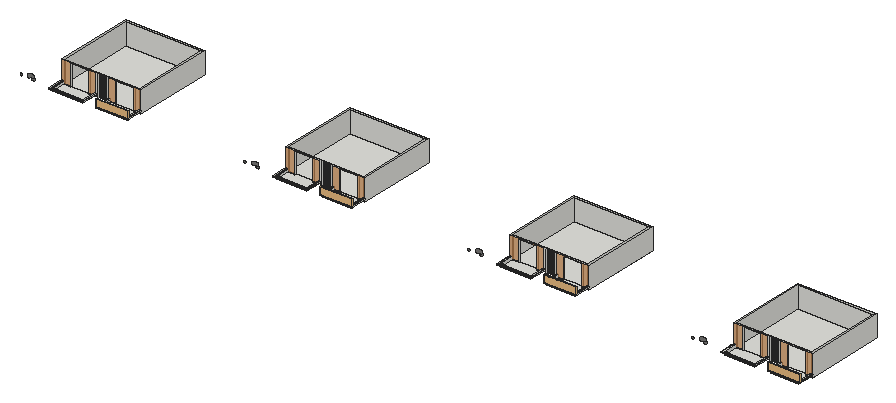
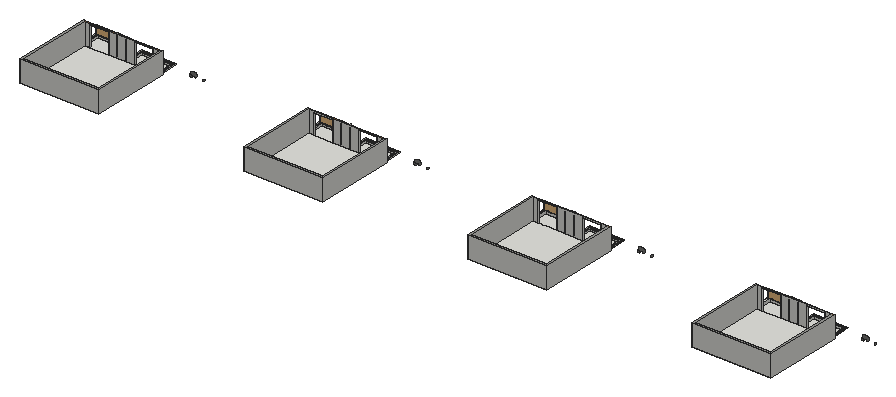
# SketchUp Ruby script. Lengths in inches.
U = 1.inch
M = Sketchup.active_model
def pt(a) = Geom::Point3d.new(a.map { |v| v * U })
def face(e, loops, mat)
  f = e.add_face(loops[0].map { |a| pt(a) })
  loops[1..].each { |l| e.add_face(l.map { |a| pt(a) }).erase! }
  f.material = f.back_material = mat if mat
  f
end
# faces: each face lists its corners as indices into pts; further lists are holes
def faces(e, pts, list, mat = nil) = list.each { |f| face(e, (f[0].is_a?(Array) ? f : [f]).map { |l| l.map { |i| pts[i] } }, mat) }
# xy, xz, yz: faces in a plane at the given z, y or x. An outline is a flat list of corners, or four numbers for a rectangle; further outlines are holes
def ring(l) = l.size == 4 ? [[l[0], l[1]], [l[2], l[1]], [l[2], l[3]], [l[0], l[3]]] : l.each_slice(2).to_a
def flat(e, list, mat, &to3) = list.each { |f| face(e, (f[0].is_a?(Array) ? f : [f]).map { |l| ring(l).map { |u, v| to3.(u, v) } }, mat) }
def xy(e, z, list, mat = nil) = flat(e, list, mat) { |x, y| [x, y, z] }
def xz(e, y, list, mat = nil) = flat(e, list, mat) { |x, z| [x, y, z] }
def yz(e, x, list, mat = nil) = flat(e, list, mat) { |y, z| [x, y, z] }
def lines(e, pts, list) = list.each { |a, b| e.add_line(pt(pts[a]), pt(pts[b])) }
# prism: a flat outline (further loops are holes) pulled along v
def prism(e, loops, v, mat = nil)
  f = face(e, loops, mat); d = Geom::Vector3d.new(v.map { |x| x * U })
  f.pushpull(f.normal.samedirection?(d) ? d.length : -d.length)
end
def box(e, o, s, mat = nil) = prism(e, [[o, [o[0] + s[0], o[1], o[2]], [o[0] + s[0], o[1] + s[1], o[2]], [o[0], o[1] + s[1], o[2]]]], [0, 0, s[2]], mat)
def at(x, y, z, deg = 0) = Geom::Transformation.translation(pt([x, y, z])) * Geom::Transformation.rotation(ORIGIN, Z_AXIS, deg.degrees)
def axes(o, x, y, z) = Geom::Transformation.new([*x, 0, *y, 0, *z, 0, *pt(o).to_a, 1])
def part(name) = M.definitions.add(name)
# library, detail: a bought-in or finely detailed component or shape, given as its bounding box
def library(name, o, s) = part(name).tap { |d| box(d.entities, o, s) }
def detail(e, o, s) = box(e.add_group.entities, o, s)
def put(e, d, t, mat = nil) = e.add_instance(d, t).tap { |i| i.material = mat if mat }
def group(e, t, mat = nil) = e.add_group.tap { |g| g.transformation = t; g.material = mat if mat }.entities
root = M.entities
M.materials.add("[0043_SaddleBrown]4").color = [124, 123, 122]
M.materials.add("[Granite Light Gray]").color = [149, 148, 144]
M.materials.add("[Wood Floor]").color = [224, 152, 88]
M.materials["[Wood Floor]"].alpha = 0.68
c1 = library("Glass Railing",[0,0,0],[139.5,4.76,42])
xy(root,526.4375,[[563.08,570.83,734.59,570.83,734.59,651.03,703.26,651.03,703.26,657.03,602.01,657.03,602.01,651.03,563.08,651.03],[820.97,570.83,978.86,570.83,978.86,651.03,951.01,651.03,951.01,657.03,849.76,657.03,849.76,651.03,820.97,651.03],[1813.71,570.83,1985.21,570.83,1985.21,651.03,1953.89,651.03,1953.89,657.03,1852.64,657.03,1852.64,651.03,1813.71,651.03],[2071.59,570.83,2229.49,570.83,2229.49,651.03,2201.63,651.03,2201.63,657.03,2100.38,657.03,2100.38,651.03,2071.59,651.03],[3064.33,570.83,3235.84,570.83,3235.84,651.03,3204.51,651.03,3204.51,657.03,3103.26,657.03,3103.26,651.03,3064.33,651.03],
  [3322.22,570.83,3480.11,570.83,3480.11,651.03,3452.26,651.03,3452.26,657.03,3351.01,657.03,3351.01,651.03,3322.22,651.03],[4314.96,570.83,4486.46,570.83,4486.46,651.03,4455.14,651.03,4455.14,657.03,4353.89,657.03,4353.89,651.03,4314.96,651.03],[4572.84,570.83,4730.74,570.83,4730.74,651.03,4702.88,651.03,4702.88,657.03,4601.63,657.03,4601.63,651.03,4572.84,651.03],[551.76,651.03,551.76,1096.5,990.19,1096.5,990.19,651.03,951.01,651.03,951.01,657.03,978.86,657.03,978.86,1085.17,563.08,1085.17,563.08,657.03,602.01,657.03,602.01,651.03],[1802.38,651.03,1802.38,1096.5,2240.81,1096.5,2240.81,651.03,2201.63,651.03,2201.63,657.03,2229.49,657.03,2229.49,1085.17,1813.71,1085.17,1813.71,657.03,1852.64,657.03,1852.64,651.03],
  [3053.01,651.03,3053.01,1096.5,3491.44,1096.5,3491.44,651.03,3452.26,651.03,3452.26,657.03,3480.11,657.03,3480.11,1085.17,3064.33,1085.17,3064.33,657.03,3103.26,657.03,3103.26,651.03],[4303.63,651.03,4303.63,1096.5,4742.06,1096.5,4742.06,651.03,4702.88,651.03,4702.88,657.03,4730.74,657.03,4730.74,1085.17,4314.96,1085.17,4314.96,657.03,4353.89,657.03,4353.89,651.03],[563.08,657.03,978.86,1085.17],[1813.71,657.03,2229.49,1085.17],[3064.33,657.03,3480.11,1085.17],
  [4314.96,657.03,4730.74,1085.17]])
xy(root,538.1875,[[550.01,558.125,742.44,559.875],[742.44,558.125,744.19,647.91],[814.68,558.125,991.94,559.875],[1800.63,558.125,1993.07,559.875],[1993.07,558.125,1994.82,647.91],
  [2065.31,558.125,2242.56,559.875],[3051.26,558.125,3243.69,559.875],[3243.69,558.125,3245.44,647.91],[3315.93,558.125,3493.19,559.875],[4301.88,558.125,4494.32,559.875],
  [4494.32,558.125,4496.07,647.91],[4566.56,558.125,4743.81,559.875],[550.01,559.875,551.76,640.11],[551.76,559.875,551.76,651.03,563.08,651.03,563.08,570.83,734.59,570.83,734.59,651.03,742.44,651.03,742.44,559.875],[814.68,559.875,814.89,651.03],
  [814.89,559.875,814.89,651.03,820.97,651.03,820.97,570.83,978.86,570.83,978.86,651.03,990.19,651.03,990.19,559.875],[990.19,559.875,991.94,651.03],[1800.63,559.875,1802.38,640.11],[1802.38,559.875,1802.38,651.03,1813.71,651.03,1813.71,570.83,1985.21,570.83,1985.21,651.03,1993.07,651.03,1993.07,559.875],[2065.31,559.875,2065.52,651.03],
  [2065.52,559.875,2065.52,651.03,2071.59,651.03,2071.59,570.83,2229.49,570.83,2229.49,651.03,2240.81,651.03,2240.81,559.875],[2240.81,559.875,2242.56,651.03],[3051.26,559.875,3053.01,640.11],[3053.01,559.875,3053.01,651.03,3064.33,651.03,3064.33,570.83,3235.84,570.83,3235.84,651.03,3243.69,651.03,3243.69,559.875],[3315.93,559.875,3316.14,651.03],
  [3316.14,559.875,3316.14,651.03,3322.22,651.03,3322.22,570.83,3480.11,570.83,3480.11,651.03,3491.44,651.03,3491.44,559.875],[3491.44,559.875,3493.19,651.03],[4301.88,559.875,4303.63,640.11],[4303.63,559.875,4303.63,651.03,4314.96,651.03,4314.96,570.83,4486.46,570.83,4486.46,651.03,4494.32,651.03,4494.32,559.875],[4566.56,559.875,4566.77,651.03],
  [4566.77,559.875,4566.77,651.03,4572.84,651.03,4572.84,570.83,4730.74,570.83,4730.74,651.03,4742.06,651.03,4742.06,559.875],[4742.06,559.875,4743.81,651.03]])
xz(root,558.125,[[550.01,538.1875,744.19,541.1875],[814.68,538.1875,991.94,541.1875],[1800.63,538.1875,1994.82,541.1875],[2065.31,538.1875,2242.56,541.1875],[3051.26,538.1875,3245.44,541.1875],
  [3315.93,538.1875,3493.19,541.1875],[4301.88,538.1875,4496.07,541.1875],[4566.56,538.1875,4743.81,541.1875]],"[Granite Light Gray]")
xz(root,570.83,[[563.08,526.4375,734.59,538.1875],[820.97,526.4375,978.86,538.1875],[1813.71,526.4375,1985.21,538.1875],[2071.59,526.4375,2229.49,538.1875],[3064.33,526.4375,3235.84,538.1875],
  [3322.22,526.4375,3480.11,538.1875],[4314.96,526.4375,4486.46,538.1875],[4572.84,526.4375,4730.74,538.1875],[563.08,538.1875,734.59,541.1875],[820.97,538.1875,978.86,541.1875],
  [1813.71,538.1875,1985.21,541.1875],[2071.59,538.1875,2229.49,541.1875],[3064.33,538.1875,3235.84,541.1875],[3322.22,538.1875,3480.11,541.1875],[4314.96,538.1875,4486.46,541.1875],
  [4572.84,538.1875,4730.74,541.1875]])
xz(root,589.17,[[437.09,527.94,436.99,528.61,436.83,529.26,436.62,529.92,436.35,530.5625,436.03,531.2,435.66,531.82,435.23,532.4375,434.76,533.04,434.24,533.62,433.67,534.18,433.05,534.73,432.39,535.26,434.04,535.17,435.7,535.18,437.35,535.3,438.98,535.51,440.55,535.83,442.07,536.25,443.51,536.76,444.86,537.35,446.1,538.03,447.23,538.78,448.22,539.6,449.07,540.47,449.07,529.79,448.03,529.77,447,529.73,445.96,529.66,444.9375,529.57,443.92,529.45,442.9,529.31,441.9,529.14,440.91,528.95,439.93,528.73,438.97,528.49,438.02,528.23],[1687.72,527.94,1687.61,528.61,1687.45,529.26,1687.24,529.92,1686.97,530.5625,1686.65,531.2,1686.28,531.82,1685.86,532.4375,1685.38,533.04,1684.86,533.62,1684.29,534.18,1683.68,534.73,1683.01,535.26,1684.67,535.17,1686.33,535.18,1687.98,535.3,1689.6,535.51,1691.18,535.83,1692.7,536.25,1694.14,536.76,1695.48,537.35,1696.73,538.03,1697.85,538.78,1698.84,539.6,1699.7,540.47,1699.7,529.79,1698.66,529.77,1697.62,529.73,1696.59,529.66,1695.5625,529.57,1694.54,529.45,1693.53,529.31,1692.53,529.14,1691.53,528.95,1690.56,528.73,1689.59,528.49,1688.65,528.23],[2938.34,527.94,2938.24,528.61,2938.08,529.26,2937.87,529.92,2937.6,530.5625,2937.28,531.2,2936.91,531.82,2936.48,532.4375,2936.01,533.04,2935.49,533.62,2934.92,534.18,2934.3,534.73,2933.64,535.26,2935.29,535.17,2936.95,535.18,2938.6,535.3,2940.23,535.51,2941.8,535.83,2943.32,536.25,2944.76,536.76,2946.11,537.35,2947.35,538.03,2948.48,538.78,2949.47,539.6,2950.32,540.47,2950.32,529.79,2949.28,529.77,2948.25,529.73,2947.21,529.66,2946.1875,529.57,2945.17,529.45,2944.15,529.31,2943.15,529.14,2942.16,528.95,2941.18,528.73,2940.22,528.49,2939.27,528.23],[4188.97,527.94,4188.86,528.61,4188.7,529.26,4188.49,529.92,4188.22,530.5625,4187.9,531.2,4187.53,531.82,4187.11,532.4375,4186.63,533.04,4186.11,533.62,4185.54,534.18,4184.93,534.73,4184.26,535.26,4185.92,535.17,4187.58,535.18,4189.23,535.3,4190.85,535.51,4192.43,535.83,4193.95,536.25,4195.39,536.76,4196.73,537.35,4197.98,538.03,4199.1,538.78,4200.09,539.6,4200.95,540.47,4200.95,529.79,4199.91,529.77,4198.87,529.73,4197.84,529.66,4196.8125,529.57,4195.79,529.45,4194.78,529.31,4193.78,529.14,4192.78,528.95,4191.81,528.73,4190.84,528.49,4189.9,528.23],[376.03,530.76,375.33,530.98,374.64,531.21,373.97,531.47,373.31,531.73,372.67,532.01,372.05,532.3,371.44,532.61,370.85,532.93,370.28,533.26,369.73,533.6,369.19,533.95,368.68,534.32,368.68,540.38,369.2,539.84,369.79,539.33,370.45,538.84,371.17,538.39,371.94,537.98,372.77,537.61,373.65,537.28,374.5625,537,375.51,536.76,376.49,536.57,377.49,536.43,378.51,536.35,378.09,535.93,377.71,535.5,377.36,535.06,377.05,534.6,376.78,534.14,376.55,533.67,376.36,533.19,376.21,532.71,376.11,532.23,376.04,531.74,376.01,531.25],
  [1626.65,530.76,1625.95,530.98,1625.27,531.21,1624.6,531.47,1623.94,531.73,1623.3,532.01,1622.67,532.3,1622.07,532.61,1621.48,532.93,1620.9,533.26,1620.35,533.6,1619.82,533.95,1619.31,534.32,1619.31,540.38,1619.83,539.84,1620.42,539.33,1621.07,538.84,1621.79,538.39,1622.57,537.98,1623.4,537.61,1624.27,537.28,1625.1875,537,1626.14,536.76,1627.12,536.57,1628.12,536.43,1629.13,536.35,1628.71,535.93,1628.33,535.5,1627.99,535.06,1627.68,534.6,1627.41,534.14,1627.18,533.67,1626.99,533.19,1626.84,532.71,1626.73,532.23,1626.66,531.74,1626.64,531.25],[2877.28,530.76,2876.58,530.98,2875.89,531.21,2875.22,531.47,2874.56,531.73,2873.92,532.01,2873.3,532.3,2872.69,532.61,2872.1,532.93,2871.53,533.26,2870.98,533.6,2870.44,533.95,2869.93,534.32,2869.93,540.38,2870.45,539.84,2871.04,539.33,2871.7,538.84,2872.42,538.39,2873.19,537.98,2874.02,537.61,2874.9,537.28,2875.8125,537,2876.76,536.76,2877.74,536.57,2878.74,536.43,2879.76,536.35,2879.34,535.93,2878.96,535.5,2878.61,535.06,2878.3,534.6,2878.03,534.14,2877.8,533.67,2877.61,533.19,2877.46,532.71,2877.36,532.23,2877.29,531.74,2877.26,531.25],[4127.9,530.76,4127.2,530.98,4126.52,531.21,4125.85,531.47,4125.19,531.73,4124.55,532.01,4123.92,532.3,4123.32,532.61,4122.73,532.93,4122.15,533.26,4121.6,533.6,4121.07,533.95,4120.56,534.32,4120.56,540.38,4121.08,539.84,4121.67,539.33,4122.32,538.84,4123.04,538.39,4123.82,537.98,4124.65,537.61,4125.52,537.28,4126.4375,537,4127.39,536.76,4128.37,536.57,4129.37,536.43,4130.38,536.35,4129.96,535.93,4129.58,535.5,4129.24,535.06,4128.93,534.6,4128.66,534.14,4128.43,533.67,4128.24,533.19,4128.09,532.71,4127.98,532.23,4127.91,531.74,4127.89,531.25],[416.47,534.48,415.35,535.4,414.34,536.36,413.45,537.37,412.6875,538.42,412.05,539.49,411.55,540.6,411.18,541.72,410.95,542.86,410.85,544.01,410.9,545.15,411.08,546.29,411.4,547.42,411.93,548.64,412.66,549.82,413.59,550.95,414.69,552.01,415.97,553,417.4,553.91,418.97,554.72,420.67,555.42,422.48,556.02,424.38,556.5,426.35,556.86,428.37,557.1,430.57,557.19,432.77,557.1,434.93,556.82,437.01,556.37,438.97,555.75,440.78,554.97,442.39,554.04,443.79,552.99,444.9375,551.84,445.82,550.59,446.42,549.29,446.73,547.95,446.72,546.78,446.4375,545.63,445.88,544.52,445.07,543.46,444.02,542.5,442.74,541.63,441.28,540.89,439.65,540.29,437.9,539.85,436.0625,539.56,434.17,539.44,432.28,539.5,430.81,539.68,429.4,540.01,428.11,540.48,426.95,541.07,425.97,541.77,425.1875,542.56,424.625,543.42,424.3,544.32,424.22,545.24,424.39,546.16,424.79,547.05,425.43,547.88,425.95,548.22,426.56,548.48,427.26,548.66,428,548.75,428.75,548.75,429.48,548.65,430.17,548.46,430.77,548.19,431.28,547.84,431.66,547.44,431.89,547,431.78,546.7,431.72,546.4,431.72,546.09,431.77,545.78,431.88,545.48,432.04,545.1875,432.26,544.91,432.52,544.65,432.84,544.4,433.19,544.18,433.58,543.99,434.01,543.83,435.02,543.91,435.99,544.1,436.91,544.37,437.75,544.73,438.49,545.16,439.12,545.65,439.61,546.2,439.96,546.79,440.16,547.41,440.21,548.03,440.09,548.66,439.82,549.26,439.08,550.27,438.07,551.1875,436.82,551.99,435.375,552.66,433.77,553.16,432.05,553.5,430.26,553.65,428.45,553.625,426.68,553.41,424.99,553.01,423.4375,552.45,422.05,551.74,420.6,550.73,419.38,549.62,418.41,548.41,417.7,547.14,417.27,545.82,417.125,544.48,417.27,543.14,417.7,541.82,418.41,540.55,419.38,539.34,420.6,538.23,422.05,537.22,421.69,536.92,421.31,536.64,420.9,536.36,420.48,536.1,420.03,535.85,419.57,535.61,419.09,535.39,418.6,535.18,418.09,534.98,417.5625,534.8,417.02,534.63],[1667.1,534.48,1665.98,535.4,1664.97,536.36,1664.08,537.37,1663.3125,538.42,1662.68,539.49,1662.17,540.6,1661.8,541.72,1661.57,542.86,1661.48,544.01,1661.52,545.15,1661.71,546.29,1662.03,547.42,1662.56,548.64,1663.29,549.82,1664.21,550.95,1665.32,552.01,1666.59,553,1668.02,553.91,1669.6,554.72,1671.3,555.42,1673.11,556.02,1675.01,556.5,1676.97,556.86,1678.99,557.1,1681.2,557.19,1683.4,557.1,1685.56,556.82,1687.64,556.37,1689.6,555.75,1691.4,554.97,1693.02,554.04,1694.41,552.99,1695.5625,551.84,1696.45,550.59,1697.05,549.29,1697.35,547.95,1697.35,546.78,1697.0625,545.63,1696.51,544.52,1695.7,543.46,1694.64,542.5,1693.37,541.63,1691.9,540.89,1690.28,540.29,1688.52,539.85,1686.6875,539.56,1684.8,539.44,1682.9,539.5,1681.43,539.68,1680.03,540.01,1678.73,540.48,1677.58,541.07,1676.59,541.77,1675.8125,542.56,1675.25,543.42,1674.93,544.32,1674.84,545.24,1675.01,546.16,1675.42,547.05,1676.06,547.88,1676.57,548.22,1677.19,548.48,1677.88,548.66,1678.62,548.75,1679.37,548.75,1680.11,548.65,1680.79,548.46,1681.4,548.19,1681.9,547.84,1682.28,547.44,1682.52,547,1682.4,546.7,1682.34,546.4,1682.34,546.09,1682.4,545.78,1682.5,545.48,1682.67,545.1875,1682.88,544.91,1683.15,544.65,1683.46,544.4,1683.82,544.18,1684.21,543.99,1684.63,543.83,1685.64,543.91,1686.62,544.1,1687.54,544.37,1688.38,544.73,1689.12,545.16,1689.74,545.65,1690.24,546.2,1690.59,546.79,1690.79,547.41,1690.83,548.03,1690.72,548.66,1690.45,549.26,1689.7,550.27,1688.69,551.1875,1687.45,551.99,1686,552.66,1684.39,553.16,1682.67,553.5,1680.89,553.65,1679.08,553.625,1677.31,553.41,1675.62,553.01,1674.0625,552.45,1672.68,551.74,1671.23,550.73,1670.01,549.62,1669.03,548.41,1668.32,547.14,1667.9,545.82,1667.75,544.48,1667.9,543.14,1668.32,541.82,1669.03,540.55,1670.01,539.34,1671.23,538.23,1672.68,537.22,1672.32,536.92,1671.93,536.64,1671.53,536.36,1671.1,536.1,1670.66,535.85,1670.2,535.61,1669.72,535.39,1669.22,535.18,1668.71,534.98,1668.1875,534.8,1667.65,534.63],
  [2917.72,534.48,2916.6,535.4,2915.59,536.36,2914.7,537.37,2913.9375,538.42,2913.3,539.49,2912.8,540.6,2912.43,541.72,2912.2,542.86,2912.1,544.01,2912.15,545.15,2912.33,546.29,2912.65,547.42,2913.18,548.64,2913.91,549.82,2914.84,550.95,2915.94,552.01,2917.22,553,2918.65,553.91,2920.22,554.72,2921.92,555.42,2923.73,556.02,2925.63,556.5,2927.6,556.86,2929.62,557.1,2931.82,557.19,2934.02,557.1,2936.18,556.82,2938.26,556.37,2940.22,555.75,2942.03,554.97,2943.64,554.04,2945.04,552.99,2946.1875,551.84,2947.07,550.59,2947.67,549.29,2947.98,547.95,2947.97,546.78,2947.6875,545.63,2947.13,544.52,2946.32,543.46,2945.27,542.5,2943.99,541.63,2942.53,540.89,2940.9,540.29,2939.15,539.85,2937.3125,539.56,2935.42,539.44,2933.53,539.5,2932.06,539.68,2930.65,540.01,2929.36,540.48,2928.2,541.07,2927.22,541.77,2926.4375,542.56,2925.875,543.42,2925.55,544.32,2925.47,545.24,2925.64,546.16,2926.04,547.05,2926.68,547.88,2927.2,548.22,2927.81,548.48,2928.51,548.66,2929.25,548.75,2930,548.75,2930.73,548.65,2931.42,548.46,2932.02,548.19,2932.53,547.84,2932.91,547.44,2933.14,547,2933.03,546.7,2932.97,546.4,2932.97,546.09,2933.02,545.78,2933.13,545.48,2933.29,545.1875,2933.51,544.91,2933.77,544.65,2934.09,544.4,2934.44,544.18,2934.83,543.99,2935.26,543.83,2936.27,543.91,2937.24,544.1,2938.16,544.37,2939,544.73,2939.74,545.16,2940.37,545.65,2940.86,546.2,2941.21,546.79,2941.41,547.41,2941.46,548.03,2941.34,548.66,2941.07,549.26,2940.33,550.27,2939.32,551.1875,2938.07,551.99,2936.625,552.66,2935.02,553.16,2933.3,553.5,2931.51,553.65,2929.7,553.625,2927.93,553.41,2926.24,553.01,2924.6875,552.45,2923.3,551.74,2921.85,550.73,2920.63,549.62,2919.66,548.41,2918.95,547.14,2918.52,545.82,2918.375,544.48,2918.52,543.14,2918.95,541.82,2919.66,540.55,2920.63,539.34,2921.85,538.23,2923.3,537.22,2922.94,536.92,2922.56,536.64,2922.15,536.36,2921.73,536.1,2921.28,535.85,2920.82,535.61,2920.34,535.39,2919.85,535.18,2919.34,534.98,2918.8125,534.8,2918.27,534.63],[4168.35,534.48,4167.23,535.4,4166.22,536.36,4165.33,537.37,4164.5625,538.42,4163.93,539.49,4163.42,540.6,4163.05,541.72,4162.82,542.86,4162.73,544.01,4162.77,545.15,4162.96,546.29,4163.28,547.42,4163.81,548.64,4164.54,549.82,4165.46,550.95,4166.57,552.01,4167.84,553,4169.27,553.91,4170.85,554.72,4172.55,555.42,4174.36,556.02,4176.26,556.5,4178.22,556.86,4180.24,557.1,4182.45,557.19,4184.65,557.1,4186.81,556.82,4188.89,556.37,4190.85,555.75,4192.65,554.97,4194.27,554.04,4195.66,552.99,4196.8125,551.84,4197.7,550.59,4198.3,549.29,4198.6,547.95,4198.6,546.78,4198.3125,545.63,4197.76,544.52,4196.95,543.46,4195.89,542.5,4194.62,541.63,4193.15,540.89,4191.53,540.29,4189.77,539.85,4187.9375,539.56,4186.05,539.44,4184.15,539.5,4182.68,539.68,4181.28,540.01,4179.98,540.48,4178.83,541.07,4177.84,541.77,4177.0625,542.56,4176.5,543.42,4176.18,544.32,4176.09,545.24,4176.26,546.16,4176.67,547.05,4177.31,547.88,4177.82,548.22,4178.44,548.48,4179.13,548.66,4179.87,548.75,4180.62,548.75,4181.36,548.65,4182.04,548.46,4182.65,548.19,4183.15,547.84,4183.53,547.44,4183.77,547,4183.65,546.7,4183.59,546.4,4183.59,546.09,4183.65,545.78,4183.75,545.48,4183.92,545.1875,4184.13,544.91,4184.4,544.65,4184.71,544.4,4185.07,544.18,4185.46,543.99,4185.88,543.83,4186.89,543.91,4187.87,544.1,4188.79,544.37,4189.63,544.73,4190.37,545.16,4190.99,545.65,4191.49,546.2,4191.84,546.79,4192.04,547.41,4192.08,548.03,4191.97,548.66,4191.7,549.26,4190.95,550.27,4189.94,551.1875,4188.7,551.99,4187.25,552.66,4185.64,553.16,4183.92,553.5,4182.14,553.65,4180.33,553.625,4178.56,553.41,4176.87,553.01,4175.3125,552.45,4173.93,551.74,4172.48,550.73,4171.26,549.62,4170.28,548.41,4169.57,547.14,4169.15,545.82,4169,544.48,4169.15,543.14,4169.57,541.82,4170.28,540.55,4171.26,539.34,4172.48,538.23,4173.93,537.22,4173.57,536.92,4173.18,536.64,4172.78,536.36,4172.35,536.1,4171.91,535.85,4171.45,535.61,4170.97,535.39,4170.47,535.18,4169.96,534.98,4169.4375,534.8,4168.9,534.63]],"[0043_SaddleBrown]4")
xz(root,640.11,[[550.01,538.1875,551.76,541.1875],[1800.63,538.1875,1802.38,541.1875],[3051.26,538.1875,3053.01,541.1875],[4301.88,538.1875,4303.63,541.1875]])
xz(root,647.91,[[742.44,538.1875,744.19,541.1875],[1993.07,538.1875,1994.82,541.1875],[3243.69,538.1875,3245.44,541.1875],[4494.32,538.1875,4496.07,541.1875]])
xz(root,651.03,[[551.76,526.4375,563.08,538.1875],[978.86,526.4375,990.19,538.1875],[1802.38,526.4375,1813.71,538.1875],[2229.49,526.4375,2240.81,538.1875],[3053.01,526.4375,3064.33,538.1875],
  [3480.11,526.4375,3491.44,538.1875],[4303.63,526.4375,4314.96,538.1875],[4730.74,526.4375,4742.06,538.1875],[551.76,538.1875,563.08,541.1875],[734.59,538.1875,742.44,541.1875],
  [814.68,538.1875,820.97,541.1875],[978.86,538.1875,990.19,541.1875],[990.19,538.1875,991.94,541.1875],[1802.38,538.1875,1813.71,541.1875],[1985.21,538.1875,1993.07,541.1875],
  [2065.31,538.1875,2071.59,541.1875],[2229.49,538.1875,2240.81,541.1875],[2240.81,538.1875,2242.56,541.1875],[3053.01,538.1875,3064.33,541.1875],[3235.84,538.1875,3243.69,541.1875],
  [3315.93,538.1875,3322.22,541.1875],[3480.11,538.1875,3491.44,541.1875],[3491.44,538.1875,3493.19,541.1875],[4303.63,538.1875,4314.96,541.1875],[4486.46,538.1875,4494.32,541.1875],
  [4566.56,538.1875,4572.84,541.1875],[4730.74,538.1875,4742.06,541.1875],[4742.06,538.1875,4743.81,541.1875]])
xz(root,651.03,[[563.08,526.4375,602.01,526.4375,602.01,640.875,703.26,640.875,703.26,526.4375,734.59,526.4375,734.59,541.1875,742.44,541.1875,742.44,646.4375,551.76,646.4375,551.76,541.1875,563.08,541.1875],[820.97,526.4375,849.76,526.4375,849.76,640.875,951.01,640.875,951.01,526.4375,978.86,526.4375,978.86,541.1875,990.19,541.1875,990.19,646.4375,814.89,646.4375,814.89,541.1875,820.97,541.1875],[1813.71,526.4375,1852.64,526.4375,1852.64,640.875,1953.89,640.875,1953.89,526.4375,1985.21,526.4375,1985.21,541.1875,1993.07,541.1875,1993.07,646.4375,1802.38,646.4375,1802.38,541.1875,1813.71,541.1875],[2071.59,526.4375,2100.38,526.4375,2100.38,640.875,2201.63,640.875,2201.63,526.4375,2229.49,526.4375,2229.49,541.1875,2240.81,541.1875,2240.81,646.4375,2065.52,646.4375,2065.52,541.1875,2071.59,541.1875],[3064.33,526.4375,3103.26,526.4375,3103.26,640.875,3204.51,640.875,3204.51,526.4375,3235.84,526.4375,3235.84,541.1875,3243.69,541.1875,3243.69,646.4375,3053.01,646.4375,3053.01,541.1875,3064.33,541.1875],
  [3322.22,526.4375,3351.01,526.4375,3351.01,640.875,3452.26,640.875,3452.26,526.4375,3480.11,526.4375,3480.11,541.1875,3491.44,541.1875,3491.44,646.4375,3316.14,646.4375,3316.14,541.1875,3322.22,541.1875],[4314.96,526.4375,4353.89,526.4375,4353.89,640.875,4455.14,640.875,4455.14,526.4375,4486.46,526.4375,4486.46,541.1875,4494.32,541.1875,4494.32,646.4375,4303.63,646.4375,4303.63,541.1875,4314.96,541.1875],[4572.84,526.4375,4601.63,526.4375,4601.63,640.875,4702.88,640.875,4702.88,526.4375,4730.74,526.4375,4730.74,541.1875,4742.06,541.1875,4742.06,646.4375,4566.77,646.4375,4566.77,541.1875,4572.84,541.1875]],"[Wood Floor]")
xz(root,657.03,[[563.08,526.4375,563.08,646.4375,978.86,646.4375,978.86,526.4375,951.01,526.4375,951.01,640.875,849.76,640.875,849.76,526.4375,703.26,526.4375,703.26,640.875,602.01,640.875,602.01,526.4375],[1813.71,526.4375,1813.71,646.4375,2229.49,646.4375,2229.49,526.4375,2201.63,526.4375,2201.63,640.875,2100.38,640.875,2100.38,526.4375,1953.89,526.4375,1953.89,640.875,1852.64,640.875,1852.64,526.4375],[3064.33,526.4375,3064.33,646.4375,3480.11,646.4375,3480.11,526.4375,3452.26,526.4375,3452.26,640.875,3351.01,640.875,3351.01,526.4375,3204.51,526.4375,3204.51,640.875,3103.26,640.875,3103.26,526.4375],[4314.96,526.4375,4314.96,646.4375,4730.74,646.4375,4730.74,526.4375,4702.88,526.4375,4702.88,640.875,4601.63,640.875,4601.63,526.4375,4455.14,526.4375,4455.14,640.875,4353.89,640.875,4353.89,526.4375]])
xz(root,1085.17,[[563.08,526.4375,978.86,646.4375],[1813.71,526.4375,2229.49,646.4375],[3064.33,526.4375,3480.11,646.4375],[4314.96,526.4375,4730.74,646.4375]])
xz(root,1096.5,[[551.76,526.4375,990.19,646.4375],[1802.38,526.4375,2240.81,646.4375],[3053.01,526.4375,3491.44,646.4375],[4303.63,526.4375,4742.06,646.4375]])
yz(root,550.01,[[558.125,538.1875,640.11,541.1875]])
yz(root,551.76,[[651.03,526.4375,1096.5,646.4375],[640.11,538.1875,651.03,541.1875]])
yz(root,563.08,[[570.83,526.4375,651.03,538.1875],[657.03,526.4375,1085.17,646.4375],[570.83,538.1875,651.03,541.1875]])
yz(root,602.01,[[651.03,526.4375,657.03,640.875]])
yz(root,703.26,[[651.03,526.4375,657.03,640.875]])
yz(root,734.59,[[570.83,526.4375,651.03,538.1875],[570.83,538.1875,651.03,541.1875]])
yz(root,742.44,[[647.91,538.1875,651.03,541.1875]])
yz(root,744.19,[[558.125,538.1875,647.91,541.1875]])
yz(root,755.44,[[647.91,526.4375,651.03,646.4375]])
yz(root,768.19,[[648.85,526.4375,651.03,646.4375]])
yz(root,780.32,[[648.85,526.4375,651.03,646.4375]])
yz(root,792.69,[[648.85,526.4375,651.03,646.4375]])
yz(root,805.57,[[648.85,526.4375,651.03,646.4375]])
yz(root,814.68,[[558.125,538.1875,648.85,541.1875],[648.85,538.1875,651.03,541.1875]])
yz(root,820.97,[[570.83,526.4375,651.03,538.1875],[570.83,538.1875,651.03,541.1875]])
yz(root,849.76,[[651.03,526.4375,657.03,640.875]])
yz(root,951.01,[[651.03,526.4375,657.03,640.875]])
yz(root,978.86,[[570.83,526.4375,651.03,538.1875],[657.03,526.4375,1085.17,646.4375],[570.83,538.1875,651.03,541.1875]])
yz(root,990.19,[[651.03,526.4375,1096.5,646.4375]])
yz(root,991.94,[[558.125,538.1875,651.03,541.1875]])
yz(root,1800.63,[[558.125,538.1875,640.11,541.1875]])
yz(root,1802.38,[[651.03,526.4375,1096.5,646.4375],[640.11,538.1875,651.03,541.1875]])
yz(root,1813.71,[[570.83,526.4375,651.03,538.1875],[657.03,526.4375,1085.17,646.4375],[570.83,538.1875,651.03,541.1875]])
yz(root,1852.64,[[651.03,526.4375,657.03,640.875]])
yz(root,1953.89,[[651.03,526.4375,657.03,640.875]])
yz(root,1985.21,[[570.83,526.4375,651.03,538.1875],[570.83,538.1875,651.03,541.1875]])
yz(root,1993.07,[[647.91,538.1875,651.03,541.1875]])
yz(root,1994.82,[[558.125,538.1875,647.91,541.1875]])
yz(root,2006.07,[[647.91,526.4375,651.03,646.4375]])
yz(root,2018.82,[[648.85,526.4375,651.03,646.4375]])
yz(root,2030.94,[[648.85,526.4375,651.03,646.4375]])
yz(root,2043.32,[[648.85,526.4375,651.03,646.4375]])
yz(root,2056.19,[[648.85,526.4375,651.03,646.4375]])
yz(root,2065.31,[[558.125,538.1875,648.85,541.1875],[648.85,538.1875,651.03,541.1875]])
yz(root,2071.59,[[570.83,526.4375,651.03,538.1875],[570.83,538.1875,651.03,541.1875]])
yz(root,2100.38,[[651.03,526.4375,657.03,640.875]])
yz(root,2201.63,[[651.03,526.4375,657.03,640.875]])
yz(root,2229.49,[[570.83,526.4375,651.03,538.1875],[657.03,526.4375,1085.17,646.4375],[570.83,538.1875,651.03,541.1875]])
yz(root,2240.81,[[651.03,526.4375,1096.5,646.4375]])
yz(root,2242.56,[[558.125,538.1875,651.03,541.1875]])
yz(root,3051.26,[[558.125,538.1875,640.11,541.1875]])
yz(root,3053.01,[[651.03,526.4375,1096.5,646.4375],[640.11,538.1875,651.03,541.1875]])
yz(root,3064.33,[[570.83,526.4375,651.03,538.1875],[657.03,526.4375,1085.17,646.4375],[570.83,538.1875,651.03,541.1875]])
yz(root,3103.26,[[651.03,526.4375,657.03,640.875]])
yz(root,3204.51,[[651.03,526.4375,657.03,640.875]])
yz(root,3235.84,[[570.83,526.4375,651.03,538.1875],[570.83,538.1875,651.03,541.1875]])
yz(root,3243.69,[[647.91,538.1875,651.03,541.1875]])
yz(root,3245.44,[[558.125,538.1875,647.91,541.1875]])
yz(root,3256.69,[[647.91,526.4375,651.03,646.4375]])
yz(root,3269.44,[[648.85,526.4375,651.03,646.4375]])
yz(root,3281.57,[[648.85,526.4375,651.03,646.4375]])
yz(root,3293.94,[[648.85,526.4375,651.03,646.4375]])
yz(root,3306.82,[[648.85,526.4375,651.03,646.4375]])
yz(root,3315.93,[[558.125,538.1875,648.85,541.1875],[648.85,538.1875,651.03,541.1875]])
yz(root,3322.22,[[570.83,526.4375,651.03,538.1875],[570.83,538.1875,651.03,541.1875]])
yz(root,3351.01,[[651.03,526.4375,657.03,640.875]])
yz(root,3452.26,[[651.03,526.4375,657.03,640.875]])
yz(root,3480.11,[[570.83,526.4375,651.03,538.1875],[657.03,526.4375,1085.17,646.4375],[570.83,538.1875,651.03,541.1875]])
yz(root,3491.44,[[651.03,526.4375,1096.5,646.4375]])
yz(root,3493.19,[[558.125,538.1875,651.03,541.1875]])
yz(root,4301.88,[[558.125,538.1875,640.11,541.1875]])
yz(root,4303.63,[[651.03,526.4375,1096.5,646.4375],[640.11,538.1875,651.03,541.1875]])
yz(root,4314.96,[[570.83,526.4375,651.03,538.1875],[657.03,526.4375,1085.17,646.4375],[570.83,538.1875,651.03,541.1875]])
yz(root,4353.89,[[651.03,526.4375,657.03,640.875]])
yz(root,4455.14,[[651.03,526.4375,657.03,640.875]])
yz(root,4486.46,[[570.83,526.4375,651.03,538.1875],[570.83,538.1875,651.03,541.1875]])
yz(root,4494.32,[[647.91,538.1875,651.03,541.1875]])
yz(root,4496.07,[[558.125,538.1875,647.91,541.1875]])
yz(root,4507.32,[[647.91,526.4375,651.03,646.4375]])
yz(root,4520.07,[[648.85,526.4375,651.03,646.4375]])
yz(root,4532.19,[[648.85,526.4375,651.03,646.4375]])
yz(root,4544.57,[[648.85,526.4375,651.03,646.4375]])
yz(root,4557.44,[[648.85,526.4375,651.03,646.4375]])
yz(root,4566.56,[[558.125,538.1875,648.85,541.1875],[648.85,538.1875,651.03,541.1875]])
yz(root,4572.84,[[570.83,526.4375,651.03,538.1875],[570.83,538.1875,651.03,541.1875]])
yz(root,4601.63,[[651.03,526.4375,657.03,640.875]])
yz(root,4702.88,[[651.03,526.4375,657.03,640.875]])
yz(root,4730.74,[[570.83,526.4375,651.03,538.1875],[657.03,526.4375,1085.17,646.4375],[570.83,538.1875,651.03,541.1875]])
yz(root,4742.06,[[651.03,526.4375,1096.5,646.4375]])
yz(root,4743.81,[[558.125,538.1875,651.03,541.1875]])
put(root,c1,axes([3315.93,559.875,538.1875],[1.2691,0,0],[0,1,0],[0,0,1]))
put(root,c1,axes([4566.56,559.875,538.1875],[1.2691,0,0],[0,1,0],[0,0,1]))
put(root,c1,axes([814.68,559.875,538.1875],[1.2691,0,0],[0,1,0],[0,0,1]))
put(root,c1,axes([2065.31,559.875,538.1875],[1.2691,0,0],[0,1,0],[0,0,1]))
